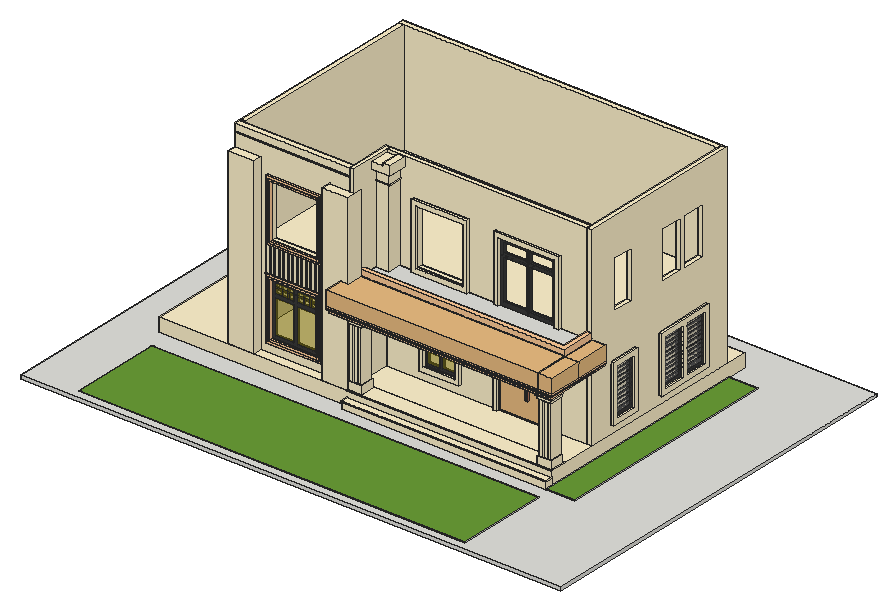
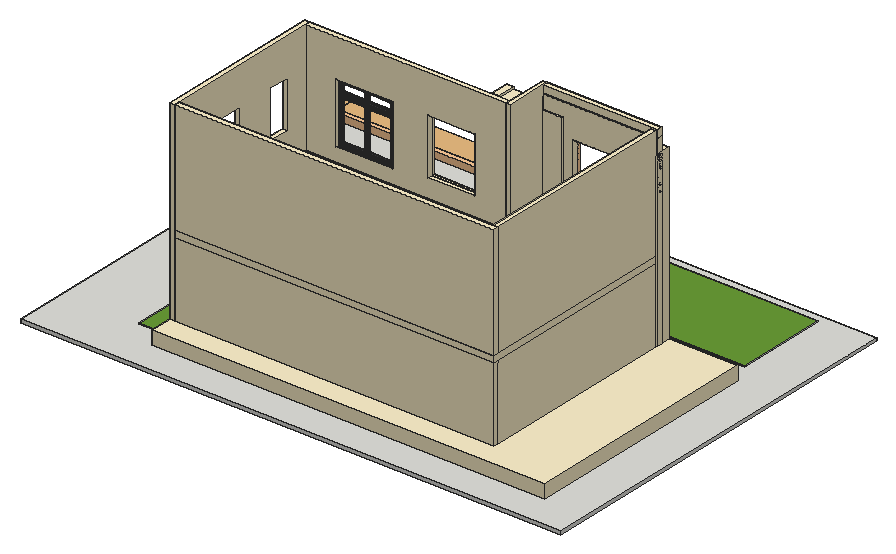
# SketchUp Ruby script. Lengths in inches.
U = 1.inch
M = Sketchup.active_model
def pt(a) = Geom::Point3d.new(a.map { |v| v * U })
def face(e, loops, mat)
  f = e.add_face(loops[0].map { |a| pt(a) })
  loops[1..].each { |l| e.add_face(l.map { |a| pt(a) }).erase! }
  f.material = f.back_material = mat if mat
  f
end
# faces: each face lists its corners as indices into pts; further lists are holes
def faces(e, pts, list, mat = nil) = list.each { |f| face(e, (f[0].is_a?(Array) ? f : [f]).map { |l| l.map { |i| pts[i] } }, mat) }
# xy, xz, yz: faces in a plane at the given z, y or x. An outline is a flat list of corners, or four numbers for a rectangle; further outlines are holes
def ring(l) = l.size == 4 ? [[l[0], l[1]], [l[2], l[1]], [l[2], l[3]], [l[0], l[3]]] : l.each_slice(2).to_a
def flat(e, list, mat, &to3) = list.each { |f| face(e, (f[0].is_a?(Array) ? f : [f]).map { |l| ring(l).map { |u, v| to3.(u, v) } }, mat) }
def xy(e, z, list, mat = nil) = flat(e, list, mat) { |x, y| [x, y, z] }
def xz(e, y, list, mat = nil) = flat(e, list, mat) { |x, z| [x, y, z] }
def yz(e, x, list, mat = nil) = flat(e, list, mat) { |y, z| [x, y, z] }
def lines(e, pts, list) = list.each { |a, b| e.add_line(pt(pts[a]), pt(pts[b])) }
# prism: a flat outline (further loops are holes) pulled along v
def prism(e, loops, v, mat = nil)
  f = face(e, loops, mat); d = Geom::Vector3d.new(v.map { |x| x * U })
  f.pushpull(f.normal.samedirection?(d) ? d.length : -d.length)
end
def box(e, o, s, mat = nil) = prism(e, [[o, [o[0] + s[0], o[1], o[2]], [o[0] + s[0], o[1] + s[1], o[2]], [o[0], o[1] + s[1], o[2]]]], [0, 0, s[2]], mat)
def at(x, y, z, deg = 0) = Geom::Transformation.translation(pt([x, y, z])) * Geom::Transformation.rotation(ORIGIN, Z_AXIS, deg.degrees)
def axes(o, x, y, z) = Geom::Transformation.new([*x, 0, *y, 0, *z, 0, *pt(o).to_a, 1])
def part(name) = M.definitions.add(name)
# library, detail: a bought-in or finely detailed component or shape, given as its bounding box
def library(name, o, s) = part(name).tap { |d| box(d.entities, o, s) }
def detail(e, o, s) = box(e.add_group.entities, o, s)
def put(e, d, t, mat = nil) = e.add_instance(d, t).tap { |i| i.material = mat if mat }
def group(e, t, mat = nil) = e.add_group.tap { |g| g.transformation = t; g.material = mat if mat }.entities
root = M.entities
M.materials.add("[Color C02]").color = [255, 204, 153]
M.materials.add("[Color D01]").color = [255, 242, 204]
M.materials.add("[Color M05]").color = [114, 114, 114]
M.materials.add("[Color M07]").color = [58, 58, 58]
M.materials.add("[Color M08]").color = [30, 30, 30]
M.materials.add("[Grass Dark Green]").color = [106, 157, 55]
M.materials.add("[Metal Rusted]").color = [184, 117, 91]
M.materials.add("[Translucent Glass Gray]").color = [128, 128, 128]
M.materials["[Translucent Glass Gray]"].alpha = 0.5
M.materials.add("[Translucent Glass Tinted]").color = [137, 125, 3]
M.materials["[Translucent Glass Tinted]"].alpha = 0.48
c1 = part("Group\#103")
box(c1.entities,[0,0,0],[45.74,28,306])
c2 = library("Group\#17",[0,-0.3,0],[112,2.3,100])
c3 = part("Group\#121")
xy(c3.entities,0,[[0,0,0,21.96,21.65,21.96,21.65,0,15.21,0,15.21,0.625,14.54,0.625,14.54,0.75,6.78,0.75,6.78,0.625,7.57,0.625,7.57,0],[6.78,0.625,14.54,0.75]])
xy(c3.entities,91.6875,[[0,0,7.57,0,7.57,0.625,6.78,0.625,6.78,0.75,14.54,0.75,14.54,0.625,15.21,0.625,15.21,0,21.65,0,21.65,21.96,0,21.96],[6.78,0.625,14.54,0.75]])
xz(c3.entities,0,[[0,0,7.57,91.6875],[15.21,0,21.65,91.6875]])
xz(c3.entities,0.625,[[6.78,0,7.57,91.6875],[7.57,0,14.54,91.6875],[14.54,0,15.21,91.6875]])
xz(c3.entities,0.75,[[6.78,0,14.54,91.6875]])
xz(c3.entities,21.96,[[0,0,21.65,91.6875]])
yz(c3.entities,0,[[0,0,21.96,91.6875]])
yz(c3.entities,6.78,[[0.625,0,0.75,91.6875]])
yz(c3.entities,7.57,[[0,0,0.625,91.6875]])
yz(c3.entities,14.54,[[0.625,0,0.75,91.6875]])
yz(c3.entities,15.21,[[0,0,0.625,91.6875]])
yz(c3.entities,21.65,[[0,0,21.96,91.6875]])
c4 = part("Group\#7")
prism(c4.entities,[[[1.17,98.4375,0.2],[1.03,98.4375,0.09],[0.87,98.4375,0.02],[0.6875,98.4375,0],[0.51,98.4375,0.02],[0.34,98.4375,0.09],[0.2,98.4375,0.2],[0.09,98.4375,0.34],[0.02,98.4375,0.51],[0,98.4375,0.6875],[0.02,98.4375,0.87],[0.09,98.4375,1.03],[0.2,98.4375,1.17],[0.34,98.4375,1.28],[0.51,98.4375,1.35],[0.6875,98.4375,1.375],[0.87,98.4375,1.35],[1.03,98.4375,1.28],[1.17,98.4375,1.17],[1.28,98.4375,1.03],[1.35,98.4375,0.87],[1.375,98.4375,0.6875],[1.35,98.4375,0.51],[1.28,98.4375,0.34]]],[0,-98.4375,0])
c5 = part("Group\#12")
prism(c5.entities,[[[1.03,0,0.09],[1.17,0,0.2],[1.28,0,0.34],[1.35,0,0.51],[1.375,0,0.6875],[1.35,0,0.87],[1.28,0,1.03],[1.17,0,1.17],[1.03,0,1.28],[0.87,0,1.35],[0.6875,0,1.375],[0.51,0,1.35],[0.34,0,1.28],[0.2,0,1.17],[0.09,0,1.03],[0.02,0,0.87],[0,0,0.6875],[0.02,0,0.51],[0.09,0,0.34],[0.2,0,0.2],[0.34,0,0.09],[0.51,0,0.02],[0.6875,0,0],[0.87,0,0.02]]],[0,35.875,0])
c6 = part("Group\#18")
prism(c6.entities,[[[0,2,20],[0,2,18.26],[0,0.74,18.26],[0,0.74,1.74],[0,2,1.74],[0,2,0],[0,0,0],[0,0,20]]],[1.99,0,0])
c7 = library("Group\#40",[-34.625,-0.5,0],[375.26,60.5,25.42])
g1 = group(root,at(487.1875,390.1875,0))
box(g1,[-487.1875,-390.1875,0],[958.5625,700.3125,6])
g2 = group(root,at(91.73,14.76,6))
xy(g2,0,[[0,0,685.3125,163.0625]])
xy(g2,1,[[0,0,685.3125,163.0625]],"[Grass Dark Green]")
xz(g2,0,[[0,0,685.3125,1]])
xz(g2,163.0625,[[0,0,685.3125,1]])
yz(g2,0,[[0,0,163.0625,1]])
yz(g2,685.3125,[[0,0,163.0625,1]])
g3 = group(root,at(530.76,403.26,6),"[Color D01]")
box(g3,[-456.375,-188.625,0],[696.375,428.625,24])
g4 = group(root,at(408.12,202.64,6),"[Color D01]")
box(g4,[0,0,0],[362.64,12,12])
g5 = group(root,at(770.76,202.64,6))
xy(g5,0,[[0,0,51.5,405.0625]])
xy(g5,1,[[0,0,51.5,405.0625]],"[Grass Dark Green]")
xz(g5,0,[[0,0,51.5,1]])
xz(g5,405.0625,[[0,0,51.5,1]])
yz(g5,0,[[0,0,405.0625,1]])
yz(g5,51.5,[[0,0,405.0625,1]])
g6 = group(root,at(408.12,201.64,18),"[Color D01]")
box(g6,[0,0,0],[362.64,13,2])
g7 = group(root,at(761.76,392.51,30),"[Color D01]")
prism(g7,[[[9,-87.87,0],[9,211.2,0],[9,211.2,343.9375],[9,-87.87,343.9375]],[[9,116.14,193],[9,116.14,277],[9,158.4,277],[9,158.4,193]],[[9,66.88,277],[9,109.14,277],[9,109.14,193],[9,66.88,193]],[[9,116.16,108],[9,158.4,108],[9,158.4,24],[9,116.16,24]],[[9,66.88,24],[9,66.88,108],[9,109.12,108],[9,109.12,24]],[[9,-38.72,277],[9,0,277],[9,0,193],[9,-38.72,193]],[[9,-38.72,24],[9,-38.72,108],[9,0,108],[9,0,24]]],[-9,0,0])
g8 = group(root,at(564.36,304.64,30),"[Color D01]")
prism(g8,[[[-158.24,0,0],[41.28,0,0],[41.28,0,108],[144.48,0,108],[144.48,0,0],[197.4,0,0],[197.4,0,132],[-158.24,0,132]],[[-32.68,0,108],[-32.68,0,24],[-89.44,0,24],[-89.44,0,108]]],[0,9,0])
g9 = group(root,at(598.76,299.64,30),"[Color D01]")
prism(g9,[[[6.88,5,0],[0,5,0],[0,5,116],[116.96,5,116],[116.96,5,0],[110.08,5,0],[110.08,5,108],[6.88,5,108]]],[0,-5,0])
g10 = group(root,at(605.64,304.64,30),"[Color M07]")
prism(g10,[[[0,7,0],[0,7,108],[103.2,7,108],[103.2,7,0]],[[99.76,7,104],[3.44,7,104],[3.44,7,4],[99.76,7,4]]],[0,-7,0])
g11 = group(root,at(398.38,232.64,30),"[Color D01]")
box(g11,[0,0,0],[7.74,81,343.9375])
g12 = group(root,at(171.88,232.64,30),"[Color D01]")
xy(g12,0,[[23.25,0,226.5,9]])
xy(g12,24,[[88.5,0,172.5,9]])
xy(g12,120,[[88.5,0,172.5,9]])
xy(g12,180,[[88.5,0,172.5,9]])
xy(g12,276,[[88.5,0,172.5,9]])
xy(g12,330,[[23.25,-1,226.5,0],[23.25,0,226.5,9]])
xy(g12,330.5,[[23.25,-1,226.5,0],[23.25,0,226.5,9]])
xy(g12,343.9375,[[23.25,0,226.5,9]])
xz(g12,-1,[[23.25,330,226.5,330.5]])
xz(g12,0,[[[23.25,0,226.5,330],[88.5,24,172.5,120],[88.5,180,172.5,276]],[23.25,330.5,226.5,343.9375]])
xz(g12,9,[[[23.25,0,226.5,330],[88.5,24,172.5,120],[88.5,180,172.5,276]],[23.25,330,226.5,330.5],[23.25,330.5,226.5,343.9375]])
yz(g12,23.25,[[0,0,9,330],[-1,330,9,330.5],[0,330.5,9,343.9375]])
yz(g12,88.5,[[0,24,9,120],[0,180,9,276]])
yz(g12,172.5,[[0,24,9,120],[0,180,9,276]])
yz(g12,226.5,[[0,0,9,330],[-1,330,9,330.5],[0,330.5,9,343.9375]])
g13 = group(root,at(83.39,594.71,30),"[Color D01]")
box(g13,[111.75,0,0],[566.625,9,132])
put(root,c1,at(362.38,216.64,30),"[Color D01]")
put(root,c1,at(195.13,216.64,30),"[Color D01]")
g14 = group(root,at(195.13,244.64,30),"[Color D01]")
box(g14,[0,0,0],[9,350.07,132])
g15 = group(root,at(408.12,214.64,30),"[Color D01]")
box(g15,[0,-1,0],[362.64,31,2])
g16 = group(root,at(746.76,214.64,30),"[Color D01]")
box(g16,[-2,0,2],[26,24,13.6])
g17 = group(root,at(408.12,216.64,30),"[Color D01]")
box(g17,[0,0,2],[24,24,13.6])
put(root,c2,axes([609.08,302.64,34],[0.86,0,0],[0,1,0],[0,0,1]),"[Color M07]")
put(root,c3,at(746.76,216.67,45.6),"[Color D01]")
put(root,c3,at(408.12,218.67,45.6),"[Color D01]")
g18 = group(root,at(770.76,452.35,46),"[Color D01]")
prism(g18,[[[0,0,100],[0,105.6,100],[0,105.6,0],[0,0,0]],[[0,7.04,8],[0,49.28,8],[0,49.28,92],[0,7.04,92]],[[0,56.32,92],[0,56.32,8],[0,98.56,8],[0,98.56,92]]],[5,0,0])
g19 = group(root,at(770.76,346.75,46),"[Color D01]")
prism(g19,[[[5,0,0],[5,52.8,0],[5,52.8,100],[5,0,100]],[[5,7.04,8],[5,7.04,92],[5,45.76,92],[5,45.76,8]]],[-5,0,0])
g20 = group(root,at(457.72,299.64,46),"[Color D01]")
prism(g20,[[[80.84,0,100],[10.32,0,100],[10.32,0,0],[80.84,0,0]],[[73.96,0,92],[73.96,0,8],[17.2,0,8],[17.2,0,92]]],[0,5,0])
g21 = group(root,at(253.38,227.64,47),"[Color C02]")
xy(g21,0,[[0,0,98,5]])
xy(g21,3,[[3,0,95,0.5]])
xy(g21,4,[[4,0,94,0.5]])
xy(g21,7,[[7,0,91,5]])
xy(g21,103,[[7,0,91,5]])
xy(g21,106,[[4,0,94,0.5]])
xy(g21,107,[[3,0,95,0.5]])
xy(g21,110,[[0,0,98,5]])
xz(g21,0,[[[0,0,98,110],[3,3,95,107]],[[4,4,94,106],[7,7,91,103]]])
xz(g21,0.5,[[[3,3,95,107],[4,4,94,106]]])
xz(g21,5,[[[0,0,98,110],[7,7,91,103]]])
yz(g21,0,[[0,0,5,110]])
yz(g21,3,[[0,3,0.5,107]])
yz(g21,4,[[0,4,0.5,106]])
yz(g21,7,[[0,7,5,103]])
yz(g21,91,[[0,7,5,103]])
yz(g21,94,[[0,4,0.5,106]])
yz(g21,95,[[0,3,0.5,107]])
yz(g21,98,[[0,0,5,110]])
g22 = group(root,at(767.76,459.39,54),"[Color M07]")
prism(g22,[[[3,0,0],[3,42.24,0],[3,42.24,84],[3,0,84]],[[3,38.72,80],[3,38.72,4],[3,3.52,4],[3,3.52,80]]],[-3,0,0])
g23 = group(root,at(767.76,508.67,54),"[Color M07]")
prism(g23,[[[3,0,84],[3,0,0],[3,42.24,0],[3,42.24,84]],[[3,3.52,80],[3,38.72,80],[3,38.72,4],[3,3.52,4]]],[-3,0,0])
g24 = group(root,at(767.76,353.79,54),"[Color M07]")
prism(g24,[[[0,0,84],[0,38.72,84],[0,38.72,0],[0,0,0]],[[0,3.52,80],[0,3.52,4],[0,35.2,4],[0,35.2,80]]],[3,0,0])
g25 = group(root,at(474.92,304.64,54),"[Color M07]")
prism(g25,[[[0,5,84],[56.76,5,84],[56.76,5,0],[0,5,0]],[[4.3,5,5],[26.23,5,5],[26.23,5,56],[4.3,5,56]],[[52.46,5,5],[52.46,5,56],[30.53,5,56],[30.53,5,5]],[[30.53,5,61],[52.46,5,61],[52.46,5,79],[30.53,5,79]],[[4.3,5,61],[26.23,5,61],[26.23,5,79],[4.3,5,79]]],[0,-5,0])
g26 = group(root,at(260.38,232.64,54),"[Color M07]")
xy(g26,0,[[0,0,84,4]])
xy(g26,6,[[6,0,39,4],[45,0,78,4]])
xy(g26,66,[[6,0,39,4],[45,0,78,4]])
xy(g26,72,[[6,0,39,4],[45,0,78,4]])
xy(g26,90,[[6,0,39,4],[45,0,78,4]])
xy(g26,96,[[0,0,84,4]])
xz(g26,0,[[[0,0,84,96],[45,6,45,66,78,66,78,72,45,72,45,90,78,90,78,6],[6,6,39,66],[6,72,39,90]]])
xz(g26,4,[[[0,0,84,96],[45,6,78,6,78,90,45,90,45,72,78,72,78,66,45,66],[6,6,39,66],[6,72,39,90]]])
yz(g26,0,[[0,0,4,96]])
yz(g26,6,[[0,6,4,66],[0,72,4,90]])
yz(g26,39,[[0,6,4,66],[0,72,4,90]])
yz(g26,45,[[0,6,4,66],[0,72,4,90]])
yz(g26,78,[[0,6,4,66],[0,66,4,72],[0,72,4,90]])
yz(g26,84,[[0,0,4,96]])
g27 = group(root,at(770.76,512.19,58),"[Translucent Glass Gray]")
yz(g27,0,[[0,0,35.2,76]])
g28 = group(root,at(770.76,462.91,58),"[Translucent Glass Gray]")
yz(g28,0,[[0,0,35.2,76]])
g29 = group(root,at(770.76,357.31,58),"[Translucent Glass Gray]")
yz(g29,0,[[0,0,31.68,76]])
g30 = group(root,at(479.22,304.64,59),"[Translucent Glass Tinted]")
xz(g30,0,[[0,0,21.93,51]])
g31 = group(root,at(505.45,304.64,59),"[Translucent Glass Tinted]")
xz(g31,0,[[0,0,21.93,51]])
g32 = group(root,at(305.38,232.64,60),"[Translucent Glass Tinted]")
xz(g32,0,[[0,0,33,60]])
g33 = group(root,at(266.38,232.64,60),"[Translucent Glass Tinted]")
xz(g33,0,[[0,0,33,60]])
put(root,c4,axes([768.57,462.91,63.73],[1,0,0],[0,0.88,0],[0,0,1]),"[Color M08]")
put(root,c5,axes([768.57,357.31,63.99],[1,0,0],[0,0.88,0],[0,0,1]),"[Color M08]")
put(root,c6,axes([654.23,300.64,64],[0.86,0,0],[0,1,0],[0,0,1]),"[Metal Rusted]")
put(root,c6,axes([658.91,300.64,64],[0.86,0,0],[0,1,0],[0,0,1]),"[Metal Rusted]")
put(root,c4,axes([768.57,462.91,70.73],[1,0,0],[0,0.88,0],[0,0,1]),"[Color M08]")
put(root,c5,axes([768.57,357.31,70.99],[1,0,0],[0,0.88,0],[0,0,1]),"[Color M08]")
put(root,c4,axes([768.57,462.91,77.73],[1,0,0],[0,0.88,0],[0,0,1]),"[Color M08]")
put(root,c5,axes([768.57,357.31,77.99],[1,0,0],[0,0.88,0],[0,0,1]),"[Color M08]")
put(root,c4,axes([768.57,462.91,84.73],[1,0,0],[0,0.88,0],[0,0,1]),"[Color M08]")
put(root,c5,axes([768.57,357.31,84.99],[1,0,0],[0,0.88,0],[0,0,1]),"[Color M08]")
put(root,c4,axes([768.57,462.91,91.73],[1,0,0],[0,0.88,0],[0,0,1]),"[Color M08]")
put(root,c5,axes([768.57,357.31,91.99],[1,0,0],[0,0.88,0],[0,0,1]),"[Color M08]")
put(root,c4,axes([768.57,462.91,98.73],[1,0,0],[0,0.88,0],[0,0,1]),"[Color M08]")
put(root,c5,axes([768.57,357.31,98.99],[1,0,0],[0,0.88,0],[0,0,1]),"[Translucent Glass Gray]")
put(root,c4,axes([768.57,462.91,105.73],[1,0,0],[0,0.88,0],[0,0,1]),"[Color M08]")
put(root,c5,axes([768.57,357.31,105.99],[1,0,0],[0,0.88,0],[0,0,1]),"[Color M08]")
put(root,c4,axes([768.57,462.91,112.73],[1,0,0],[0,0.88,0],[0,0,1]),"[Color M08]")
put(root,c5,axes([768.57,357.31,112.99],[1,0,0],[0,0.88,0],[0,0,1]),"[Color M08]")
g34 = group(root,at(519.86,306.14,115),"[Color M08]")
prism(g34,[[[1.08,1.97,0],[1.29,1.87,0],[1.47,1.71,0],[1.6,1.5,0],[1.69,1.26,0],[1.72,1,0],[1.69,0.74,0],[1.6,0.5,0],[1.47,0.29,0],[1.29,0.13,0],[1.08,0.03,0],[0.86,0,0],[0.64,0.03,0],[0.43,0.13,0],[0.25,0.29,0],[0.12,0.5,0],[0.03,0.74,0],[0,1,0],[0.03,1.26,0],[0.12,1.5,0],[0.25,1.71,0],[0.43,1.87,0],[0.64,1.97,0],[0.86,2,0]]],[0,0,18])
g35 = group(root,at(511.26,306.14,115),"[Color M08]")
prism(g35,[[[0,0.95,0],[0.02,1.21,0],[0.09,1.46,0],[0.22,1.67,0],[0.39,1.84,0],[0.6,1.95,0],[0.82,2,0],[1.04,1.98,0],[1.25,1.89,0],[1.4375,1.74,0],[1.58,1.54,0],[1.68,1.3,0],[1.72,1.05,0],[1.7,0.79,0],[1.625,0.54,0],[1.5,0.33,0],[1.32,0.16,0],[1.12,0.05,0],[0.9,0,0],[0.68,0.02,0],[0.47,0.11,0],[0.28,0.26,0],[0.14,0.46,0],[0.04,0.69,0]]],[0,0,17.9375])
g36 = group(root,at(493.63,306.14,115),"[Color M08]")
prism(g36,[[[1.47,0.29,0],[1.29,0.13,0],[1.08,0.03,0],[0.86,0,0],[0.64,0.03,0],[0.43,0.13,0],[0.25,0.29,0],[0.12,0.5,0],[0.03,0.74,0],[0,1,0],[0.03,1.26,0],[0.12,1.5,0],[0.25,1.71,0],[0.43,1.87,0],[0.64,1.97,0],[0.86,2,0],[1.08,1.97,0],[1.29,1.87,0],[1.47,1.71,0],[1.6,1.5,0],[1.69,1.26,0],[1.72,1,0],[1.69,0.74,0],[1.6,0.5,0]]],[0,0,18])
g37 = group(root,at(485.03,306.14,115),"[Color M08]")
prism(g37,[[[0.64,1.97,0],[0.86,2,0],[1.08,1.97,0],[1.29,1.87,0],[1.47,1.71,0],[1.6,1.5,0],[1.69,1.26,0],[1.72,1,0],[1.69,0.74,0],[1.6,0.5,0],[1.47,0.29,0],[1.29,0.13,0],[1.08,0.03,0],[0.86,0,0],[0.64,0.03,0],[0.43,0.13,0],[0.25,0.29,0],[0.12,0.5,0],[0.03,0.74,0],[0,1,0],[0.03,1.26,0],[0.12,1.5,0],[0.25,1.71,0],[0.43,1.87,0]]],[0,0,18])
g38 = group(root,at(479.22,304.64,115),"[Translucent Glass Tinted]")
xz(g38,0,[[0,0,21.93,18]])
g39 = group(root,at(505.45,304.64,115),"[Translucent Glass Tinted]")
xz(g39,0,[[0,0,21.93,18]])
put(root,c4,axes([768.57,462.91,119.73],[1,0,0],[0,0.88,0],[0,0,1]),"[Color M08]")
put(root,c5,axes([768.57,357.31,119.99],[1,0,0],[0,0.88,0],[0,0,1]),"[Color M08]")
g40 = group(root,at(479.22,306.14,123),"[Color M08]")
prism(g40,[[[0,1.5,0.13],[0,1.26,0.03],[0,1,0],[0,0.74,0.03],[0,0.5,0.13],[0,0.29,0.29],[0,0.13,0.5],[0,0.03,0.74],[0,0,1],[0,0.03,1.26],[0,0.13,1.5],[0,0.29,1.71],[0,0.5,1.87],[0,0.74,1.97],[0,1,2],[0,1.26,1.97],[0,1.5,1.87],[0,1.71,1.71],[0,1.87,1.5],[0,1.97,1.26],[0,2,1],[0,1.97,0.74],[0,1.87,0.5],[0,1.71,0.29]]],[48.16,0,0])
g41 = group(root,at(275.89,233.64,126),"[Color M08]")
prism(g41,[[[1.57,0.18,0],[1.34,0.06,0],[1.08,0,0],[0.82,0.01,0],[0.57,0.09,0],[0.35,0.23,0],[0.18,0.42,0],[0.06,0.65,0],[0,0.91,0],[0.01,1.17,0],[0.09,1.42,0],[0.23,1.64,0],[0.42,1.82,0],[0.65,1.9375,0],[0.91,1.99,0],[1.17,1.98,0],[1.42,1.9,0],[1.64,1.76,0],[1.82,1.57,0],[1.9375,1.34,0],[1.99,1.08,0],[1.98,0.82,0],[1.9,0.57,0],[1.76,0.35,0]]],[0,0,18])
g42 = group(root,at(287.88,233.64,126),"[Color M08]")
prism(g42,[[[2,1,0],[1.97,0.74,0],[1.87,0.5,0],[1.71,0.29,0],[1.5,0.13,0],[1.26,0.03,0],[1,0,0],[0.74,0.03,0],[0.5,0.13,0],[0.29,0.29,0],[0.13,0.5,0],[0.03,0.74,0],[0,1,0],[0.03,1.26,0],[0.13,1.5,0],[0.29,1.71,0],[0.5,1.87,0],[0.74,1.97,0],[1,2,0],[1.26,1.97,0],[1.5,1.87,0],[1.71,1.71,0],[1.87,1.5,0],[1.97,1.26,0]]],[0,0,18])
g43 = group(root,at(314.88,233.64,126),"[Color M08]")
prism(g43,[[[1.5,0.13,0],[1.26,0.03,0],[1,0,0],[0.74,0.03,0],[0.5,0.13,0],[0.29,0.29,0],[0.13,0.5,0],[0.03,0.74,0],[0,1,0],[0.03,1.26,0],[0.13,1.5,0],[0.29,1.71,0],[0.5,1.87,0],[0.74,1.97,0],[1,2,0],[1.26,1.97,0],[1.5,1.87,0],[1.71,1.71,0],[1.87,1.5,0],[1.97,1.26,0],[2,1,0],[1.97,0.74,0],[1.87,0.5,0],[1.71,0.29,0]]],[0,0,18])
g44 = group(root,at(326.88,233.64,126),"[Color M08]")
prism(g44,[[[2,1,0],[1.97,0.74,0],[1.87,0.5,0],[1.71,0.29,0],[1.5,0.13,0],[1.26,0.03,0],[1,0,0],[0.74,0.03,0],[0.5,0.13,0],[0.29,0.29,0],[0.13,0.5,0],[0.03,0.74,0],[0,1,0],[0.03,1.26,0],[0.13,1.5,0],[0.29,1.71,0],[0.5,1.87,0],[0.74,1.97,0],[1,2,0],[1.26,1.97,0],[1.5,1.87,0],[1.71,1.71,0],[1.87,1.5,0],[1.97,1.26,0]]],[0,0,18])
g45 = group(root,at(266.38,232.64,126),"[Translucent Glass Tinted]")
xz(g45,0,[[0,0,33,18]])
g46 = group(root,at(305.38,232.64,126),"[Translucent Glass Tinted]")
xz(g46,0,[[0,0,33,18]])
put(root,c4,axes([768.57,462.91,126.73],[1,0,0],[0,0.88,0],[0,0,1]),"[Color M08]")
put(root,c5,axes([768.57,357.31,126.99],[1,0,0],[0,0.88,0],[0,0,1]),"[Color M08]")
g47 = group(root,at(266.38,233.64,134),"[Color M08]")
prism(g47,[[[0,0.74,0.03],[0,0.5,0.13],[0,0.29,0.29],[0,0.13,0.5],[0,0.03,0.74],[0,0,1],[0,0.03,1.26],[0,0.13,1.5],[0,0.29,1.71],[0,0.5,1.87],[0,0.74,1.97],[0,1,2],[0,1.26,1.97],[0,1.5,1.87],[0,1.71,1.71],[0,1.87,1.5],[0,1.97,1.26],[0,2,1],[0,1.97,0.74],[0,1.87,0.5],[0,1.71,0.29],[0,1.5,0.13],[0,1.26,0.03],[0,1,0]]],[72,0,0])
g48 = group(root,at(746.76,214.67,137.29),"[Color D01]")
box(g48,[-2,0,0],[25.65,23.96,5])
g49 = group(root,at(408.12,216.67,137.29),"[Color D01]")
box(g49,[0,0,0],[23.65,23.96,5])
g50 = group(root,at(746.76,212.67,142.29),"[Color D01]")
box(g50,[-4,0,0],[29.65,25.96,6])
g51 = group(root,at(408.12,214.67,142.29),"[Color D01]")
box(g51,[0,0,0],[25.65,25.96,6])
g52 = group(root,at(746.76,209.67,148.29),"[Color D01]")
box(g52,[-7,0,0],[35.65,28.96,7.71])
g53 = group(root,at(408.12,211.67,148.29),"[Color D01]")
box(g53,[0,0,0],[28.65,28.96,7.71])
g54 = group(root,at(406.12,208.64,156))
box(g54,[-7.74,0,0],[372.38,96,18])
g55 = group(root,at(394.12,184.64,156),"[Color C02]")
xy(g55,0,[[0,18,0,24,376.64,24,376.64,120,382.64,120,382.64,18]])
xy(g55,2,[[0,16,0,18,382.64,18,382.64,120,384.64,120,384.64,16]])
xy(g55,4,[[0,7,0,16,384.64,16,384.64,120,393.64,120,393.64,7]])
xy(g55,10,[[0,2,0,7,393.64,7,393.64,120,398.64,120,398.64,2]])
xy(g55,13,[[0,0,0,2,398.64,2,398.64,120,400.64,120,400.64,0]])
xy(g55,14,[[0,0,400.64,0,400.64,120,399.64,120,399.64,1,0,1]])
xy(g55,15,[[0,0,0,1,399.64,1,399.64,120,400.64,120,400.64,0]])
xy(g55,18,[[0,0,400.64,0,400.64,120,376.64,120,376.64,24,0,24]])
xz(g55,0,[[0,13,400.64,14],[0,15,400.64,18]])
xz(g55,1,[[0,14,399.64,15]])
xz(g55,2,[[0,10,398.64,13]])
xz(g55,7,[[0,4,393.64,10]])
xz(g55,16,[[0,2,384.64,4]])
xz(g55,18,[[0,0,382.64,2]])
xz(g55,24,[[0,0,376.64,9],[0,9,376.64,18]])
xz(g55,120,[[376.64,0,376.64,18,400.64,18,400.64,15,399.64,15,399.64,14,400.64,14,400.64,13,398.64,13,398.64,10,393.64,10,393.64,4,384.64,4,384.64,2,382.64,2,382.64,0]])
yz(g55,0,[[18,0,18,2,16,2,16,4,7,4,7,10,2,10,2,13,0,13,0,14,1,14,1,15,0,15,0,18,24,18,24,0]])
yz(g55,376.64,[[24,0,120,9],[24,9,120,18]])
yz(g55,382.64,[[18,0,120,2]])
yz(g55,384.64,[[16,2,120,4]])
yz(g55,393.64,[[7,4,120,10]])
yz(g55,398.64,[[2,10,120,13]])
yz(g55,399.64,[[1,14,120,15]])
yz(g55,400.64,[[0,13,120,14],[0,15,120,18]])
g56 = group(root,at(252.38,227.64,157))
box(g56,[0,0,0],[100,5,1])
g57 = group(root,at(253.38,230.64,158),"[Color D01]")
xy(g57,0,[[0,-2,0,2,7.5,2,7.5,0,6,0,6,-2],[7.5,-2,14,2],[15.5,-2,15.5,0,14,0,14,2,99,2,99,-2,95.5,-2,95.5,0,94,0,94,-2,87.5,-2,87.5,0,86,0,86,-2,79.5,-2,79.5,0,78,0,78,-2,71.5,-2,71.5,0,70,0,70,-2,63.5,-2,63.5,0,62,0,62,-2,55.5,-2,55.5,0,54,0,54,-2,47.5,-2,47.5,0,46,0,46,-2,39.5,-2,39.5,0,38,0,38,-2,31.5,-2,31.5,0,30,0,30,-2,23.5,-2,23.5,0,22,0,22,-2]])
xy(g57,45,[[0,-2,6,-2,6,0,7.5,0,7.5,2,0,2],[7.5,-2,14,2],[15.5,-2,22,-2,22,0,23.5,0,23.5,-2,30,-2,30,0,31.5,0,31.5,-2,38,-2,38,0,39.5,0,39.5,-2,46,-2,46,0,47.5,0,47.5,-2,54,-2,54,0,55.5,0,55.5,-2,62,-2,62,0,63.5,0,63.5,-2,70,-2,70,0,71.5,0,71.5,-2,78,-2,78,0,79.5,0,79.5,-2,86,-2,86,0,87.5,0,87.5,-2,94,-2,94,0,95.5,0,95.5,-2,99,-2,99,2,14,2,14,0,15.5,0]])
xz(g57,-2,[[0,0,6,45],[7.5,0,14,45],[15.5,0,22,45],[23.5,0,30,45],[31.5,0,38,45],
  [39.5,0,46,45],[47.5,0,54,45],[55.5,0,62,45],[63.5,0,70,45],[71.5,0,78,45],
  [79.5,0,86,45],[87.5,0,94,45],[95.5,0,99,45]])
xz(g57,0,[[6,0,7.5,45],[14,0,15.5,45],[22,0,23.5,45],[30,0,31.5,45],[38,0,39.5,45],
  [46,0,47.5,45],[54,0,55.5,45],[62,0,63.5,45],[70,0,71.5,45],[78,0,79.5,45],
  [86,0,87.5,45],[94,0,95.5,45]])
xz(g57,2,[[0,0,7.5,45],[7.5,0,14,45],[14,0,99,45]])
yz(g57,0,[[-2,0,2,45]])
yz(g57,6,[[-2,0,0,45]])
yz(g57,7.5,[[-2,0,0,45],[0,0,2,45]])
yz(g57,14,[[-2,0,0,45],[0,0,2,45]])
yz(g57,15.5,[[-2,0,0,45]])
yz(g57,22,[[-2,0,0,45]])
yz(g57,23.5,[[-2,0,0,45]])
yz(g57,30,[[-2,0,0,45]])
yz(g57,31.5,[[-2,0,0,45]])
yz(g57,38,[[-2,0,0,45]])
yz(g57,39.5,[[-2,0,0,45]])
yz(g57,46,[[-2,0,0,45]])
yz(g57,47.5,[[-2,0,0,45]])
yz(g57,54,[[-2,0,0,45]])
yz(g57,55.5,[[-2,0,0,45]])
yz(g57,62,[[-2,0,0,45]])
yz(g57,63.5,[[-2,0,0,45]])
yz(g57,70,[[-2,0,0,45]])
yz(g57,71.5,[[-2,0,0,45]])
yz(g57,78,[[-2,0,0,45]])
yz(g57,79.5,[[-2,0,0,45]])
yz(g57,86,[[-2,0,0,45]])
yz(g57,87.5,[[-2,0,0,45]])
yz(g57,94,[[-2,0,0,45]])
yz(g57,95.5,[[-2,0,0,45]])
yz(g57,99,[[-2,0,2,45]])
g58 = group(root,at(74.39,304.64,162),"[Color D01]")
prism(g58,[[[687.375,299.07,0],[687.375,0,0],[323.99,0,0],[323.99,-60,0],[120.75,-60,0],[120.75,299.07,0]]],[0,0,12])
g59 = group(root,at(195.13,594.71,174),"[Color D01]")
box(g59,[0,0,0],[566.63,9,199.9375])
g60 = group(root,at(195.13,244.64,174),"[Color D01]")
box(g60,[0,0,0],[9,350.07,199.9375])
g61 = group(root,at(406.12,304.64,174),"[Color D01]")
prism(g61,[[[0,0,0],[355.64,0,0],[355.64,0,199.9375],[0,0,199.9375]],[[301.64,0,24],[201.64,0,24],[201.64,0,132],[301.64,0,132]],[[55.92,0,132],[138.44,0,132],[138.44,0,32],[55.92,0,32]]],[0,9,0])
g62 = group(root,at(430.12,244.64,174))
box(g62,[-24,0,0],[364.64,60,24])
put(root,c7,at(430.12,184.64,174),"[Color M05]")
g63 = group(root,at(770.76,244.64,174),"[Color M05]")
detail(g63,[0,0,0],[24.99,60,25.13])
g64 = group(root,at(770.76,184.64,174),"[Color M05]")
detail(g64,[0,0,0],[24,60,24.51])
g65 = group(root,at(770.76,184.64,174),"[Color M05]")
p = [[18.0625,16.1,8.2],[17.58,16.1,8.62],[8.65,38.4,16.43],[9.03,38.4,16.1]]
lines(g65,p,[[0,1],[2,3]])
detail(g65,[0,0,0],[24.99,60,25.13])
g66 = group(root,at(599.76,299.64,198),"[Color D01]")
prism(g66,[[[0,0,0],[8,0,0],[8,0,108],[108,0,108],[108,0,0],[116,0,0],[116,0,116],[0,0,116]]],[0,5,0])
g67 = group(root,at(607.76,304.14,198),"[Color M07]")
xy(g67,0,[[0,0,0,5,100,5,100,0,50.15,0,50.15,0.5,49.85,0.5,49.85,0]])
xy(g67,6,[[6,0,47,5],[53,0,94,5]])
xy(g67,78,[[6,0,47,5],[53,0,94,5]])
xy(g67,80.85,[[3,0,49.85,0.5],[50.15,0,97,0.5]])
xy(g67,81.15,[[3,0,49.85,0.5],[50.15,0,97,0.5]])
xy(g67,84,[[6,0,47,5],[53,0,94,5]])
xy(g67,102,[[6,0,47,5],[53,0,94,5]])
xy(g67,108,[[0,0,49.85,0,49.85,0.5,50.15,0.5,50.15,0,100,0,100,5,0,5]])
xz(g67,0,[[[0,0,49.85,0,49.85,80.85,3,80.85,3,81.15,49.85,81.15,49.85,108,0,108],[6,6,47,78],[6,84,47,102]],[[50.15,0,100,0,100,108,50.15,108,50.15,81.15,97,81.15,97,80.85,50.15,80.85],[53,6,94,78],[53,84,94,102]]])
xz(g67,0.5,[[49.85,0,50.15,0,50.15,80.85,97,80.85,97,81.15,50.15,81.15,50.15,108,49.85,108,49.85,81.15,3,81.15,3,80.85,49.85,80.85]])
xz(g67,5,[[[0,0,100,108],[6,6,47,78],[53,6,94,78],[6,84,47,102],[53,84,94,102]]])
yz(g67,0,[[0,0,5,108]])
yz(g67,3,[[0,80.85,0.5,81.15]])
yz(g67,6,[[0,6,5,78],[0,84,5,102]])
yz(g67,47,[[0,6,5,78],[0,84,5,102]])
yz(g67,49.85,[[0,0,0.5,80.85],[0,81.15,0.5,108]])
yz(g67,50.15,[[0,0,0.5,80.85],[0,81.15,0.5,108]])
yz(g67,53,[[0,6,5,78],[0,84,5,102]])
yz(g67,94,[[0,6,5,78],[0,84,5,102]])
yz(g67,97,[[0,80.85,0.5,81.15]])
yz(g67,100,[[0,0,5,108]])
g68 = group(root,at(454.04,299.64,198),"[Color D01]")
prism(g68,[[[98.52,0,0],[98.52,0,116],[0,0,116],[0,0,0]],[[90.52,0,108],[90.52,0,8],[8,0,8],[8,0,108]]],[0,5,0])
g69 = group(root,at(406.12,279.64,198),"[Color D01]")
xy(g69,0,[[0,1,24,25]])
xy(g69,138,[[0,0,25,1],[0,1,24,25],[24,1,25,25]])
xy(g69,139,[[0,0,25,1],[0,1,24,25],[24,1,25,25]])
xy(g69,159.46,[[0,0,25,1],[0,1,24,25],[24,1,25,25]])
xy(g69,159.96,[[0,-9,33,0],[0,0,25,25],[25,0,33,1],[25,1,33,25]])
xy(g69,172.25,[[0,-9,20.26,25]])
xy(g69,175.9375,[[20.26,-9,33,25]])
xz(g69,-9,[[0,159.96,33,159.96,33,175.9375,20.26,175.9375,20.26,172.25,0,172.25]])
xz(g69,0,[[0,138,25,139],[0,159.46,25,159.96]])
xz(g69,1,[[0,0,24,138],[0,139,24,159.46]])
xz(g69,25,[[0,0,24,138],[0,138,25,139],[0,139,24,159.46],[0,159.46,25,159.96],[0,159.96,0,172.25,20.26,172.25,20.26,175.9375,33,175.9375,33,159.96]])
yz(g69,0,[[1,0,25,138],[0,138,25,139],[1,139,25,159.46],[0,159.46,25,159.96],[-9,159.96,25,172.25]])
yz(g69,20.26,[[-9,172.25,25,175.9375]])
yz(g69,24,[[1,0,25,138],[1,139,25,159.46]])
yz(g69,25,[[0,138,25,139],[0,159.46,25,159.96]])
yz(g69,33,[[-9,159.96,25,175.9375]])
g70 = group(root,at(406.12,244.64,198),"[Color C02]")
prism(g70,[[[0,0,0],[0,9,0],[355.64,9,0],[355.64,60,0],[364.64,60,0],[364.64,0,0]]],[0,0,12])
g71 = group(root,at(253.38,227.64,203),"[Color C02]")
xy(g71,0,[[0,0,98,5]])
xy(g71,3.02,[[3.02,0,94.98,0.5]])
xy(g71,4.02,[[4.02,0,93.98,0.5]])
xy(g71,7,[[7,0,91,5]])
xy(g71,103,[[7,0,91,5]])
xy(g71,105.98,[[4.02,0,93.98,0.5]])
xy(g71,106.98,[[3.02,0,94.98,0.5]])
xy(g71,110,[[0,0,98,5]])
xz(g71,0,[[[0,0,98,110],[3.02,3.02,94.98,106.98]],[[4.02,4.02,93.98,105.98],[7,7,91,103]]])
xz(g71,0.5,[[[3.02,3.02,94.98,106.98],[4.02,4.02,93.98,105.98]]])
xz(g71,5,[[[0,0,98,110],[7,7,91,103]]])
yz(g71,0,[[0,0,5,110]])
yz(g71,3.02,[[0,3.02,0.5,106.98]])
yz(g71,4.02,[[0,4.02,0.5,105.98]])
yz(g71,7,[[0,7,5,103]])
yz(g71,91,[[0,7,5,103]])
yz(g71,93.98,[[0,4.02,0.5,105.98]])
yz(g71,94.98,[[0,3.02,0.5,106.98]])
yz(g71,98,[[0,0,5,110]])
